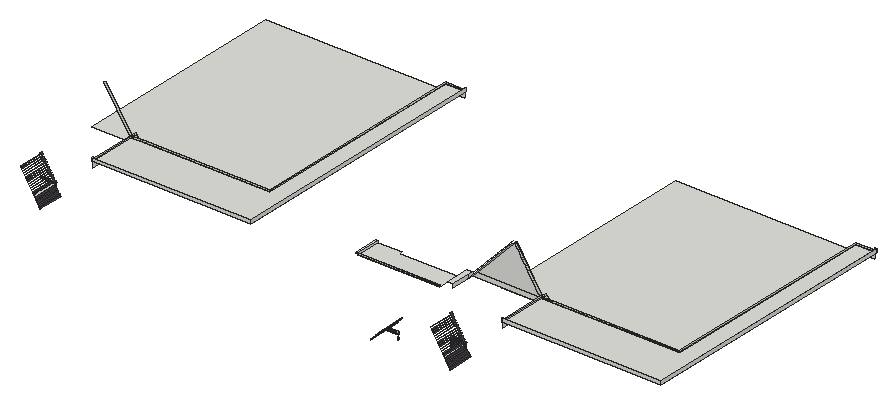
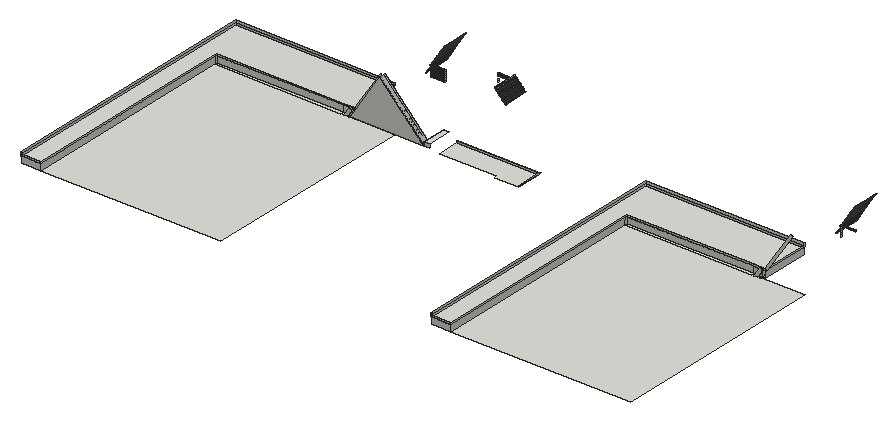
# SketchUp Ruby script. Lengths in inches.
U = 1.inch
M = Sketchup.active_model
def pt(a) = Geom::Point3d.new(a.map { |v| v * U })
def face(e, loops, mat)
  f = e.add_face(loops[0].map { |a| pt(a) })
  loops[1..].each { |l| e.add_face(l.map { |a| pt(a) }).erase! }
  f.material = f.back_material = mat if mat
  f
end
# faces: each face lists its corners as indices into pts; further lists are holes
def faces(e, pts, list, mat = nil) = list.each { |f| face(e, (f[0].is_a?(Array) ? f : [f]).map { |l| l.map { |i| pts[i] } }, mat) }
# xy, xz, yz: faces in a plane at the given z, y or x. An outline is a flat list of corners, or four numbers for a rectangle; further outlines are holes
def ring(l) = l.size == 4 ? [[l[0], l[1]], [l[2], l[1]], [l[2], l[3]], [l[0], l[3]]] : l.each_slice(2).to_a
def flat(e, list, mat, &to3) = list.each { |f| face(e, (f[0].is_a?(Array) ? f : [f]).map { |l| ring(l).map { |u, v| to3.(u, v) } }, mat) }
def xy(e, z, list, mat = nil) = flat(e, list, mat) { |x, y| [x, y, z] }
def xz(e, y, list, mat = nil) = flat(e, list, mat) { |x, z| [x, y, z] }
def yz(e, x, list, mat = nil) = flat(e, list, mat) { |y, z| [x, y, z] }
def lines(e, pts, list) = list.each { |a, b| e.add_line(pt(pts[a]), pt(pts[b])) }
# prism: a flat outline (further loops are holes) pulled along v
def prism(e, loops, v, mat = nil)
  f = face(e, loops, mat); d = Geom::Vector3d.new(v.map { |x| x * U })
  f.pushpull(f.normal.samedirection?(d) ? d.length : -d.length)
end
def box(e, o, s, mat = nil) = prism(e, [[o, [o[0] + s[0], o[1], o[2]], [o[0] + s[0], o[1] + s[1], o[2]], [o[0], o[1] + s[1], o[2]]]], [0, 0, s[2]], mat)
def at(x, y, z, deg = 0) = Geom::Transformation.translation(pt([x, y, z])) * Geom::Transformation.rotation(ORIGIN, Z_AXIS, deg.degrees)
def axes(o, x, y, z) = Geom::Transformation.new([*x, 0, *y, 0, *z, 0, *pt(o).to_a, 1])
def part(name) = M.definitions.add(name)
# library, detail: a bought-in or finely detailed component or shape, given as its bounding box
def library(name, o, s) = part(name).tap { |d| box(d.entities, o, s) }
def detail(e, o, s) = box(e.add_group.entities, o, s)
def put(e, d, t, mat = nil) = e.add_instance(d, t).tap { |i| i.material = mat if mat }
def group(e, t, mat = nil) = e.add_group.tap { |g| g.transformation = t; g.material = mat if mat }.entities
root = M.entities
M.materials.add("[Color M06]").color = [79, 71, 84]
xy(root,341.52,[[2350.98,524.25,2381.95,526.125]])
xy(root,341.93,[[2350.98,524.25,2381.95,526.125]])
xy(root,342.6875,[[2025.57,678.64,2202.51,678.64,2202.51,726.125,2079.13,726.125,2079.13,732.2,2025.57,732.2]])
xy(root,345.06,[[2350.98,524.25,2381.95,526.125]])
xy(root,346,[[2350.98,524.25,2381.95,526.125]])
xy(root,346.3125,[[2023.01,676.08,2025.57,678.64],[2025.57,676.08,2202.51,678.64],[2023.01,678.64,2025.57,732.2]])
xy(root,349.12,[[2350.98,524.25,2381.95,526.125]])
xy(root,350.06,[[2350.98,524.25,2381.95,526.125]])
xy(root,350.1875,[[1523.88,726.125,1797.03,732.2],[2410.35,726.125,2683.5,732.2],[1409.09,732.2,1797.03,1201.875],[2295.55,732.2,2683.5,1201.875]])
xy(root,353.18,[[2350.98,524.25,2381.95,526.125]])
xy(root,354.12,[[2350.98,524.25,2381.95,526.125]])
xy(root,357.25,[[2350.98,524.25,2381.95,526.125]])
xy(root,358.06,[[2350.98,524.25,2381.95,526.125]])
xy(root,358.5,[[2219.8,678.64,2232.12,732.2]])
xy(root,361.18,[[2350.98,524.25,2381.95,526.125]])
xy(root,361.84,[[2244.03,480.14,2246.29,480.77],[2246.89,480.14,2249.21,480.77],[2249.81,480.14,2252.12,480.77],[2252.72,480.14,2255.03,480.77],[2255.63,480.14,2257.94,480.77],
  [2258.54,480.14,2260.86,480.77],[2261.45,480.14,2263.77,480.77],[2264.37,480.14,2266.68,480.77],[2267.28,480.14,2269.59,480.77],[2270.19,480.14,2272.5,480.77]])
xy(root,362,[[2350.98,524.25,2381.95,526.125]])
xy(root,363.75,[[1497.82,620.41,1838.47,623.84],[1838.47,620.41,1841.91,623.84],[2384.28,620.41,2724.93,623.84],[2724.93,620.41,2728.37,623.84],[1497.82,623.84,1497.82,726.125,1797.03,726.125,1797.03,1201.875,1838.47,1201.875,1838.47,623.84],
  [1838.47,623.84,1841.91,1201.875],[2384.28,623.84,2384.28,726.125,2683.5,726.125,2683.5,1201.875,2724.93,1201.875,2724.93,623.84],[2724.93,623.84,2728.37,1201.875]])
xy(root,363.92,[[1495.49,521.5625,1497.36,526.125],[2381.95,521.5625,2383.83,526.125]])
xy(root,364.15,[[2246.2,480.14,2246.29,480.77],[2246.89,480.14,2249.21,480.77],[2249.81,480.14,2252.12,480.77],[2252.72,480.14,2255.03,480.77],[2255.63,480.14,2257.94,480.77],
  [2258.54,480.14,2260.86,480.77],[2261.45,480.14,2263.77,480.77],[2264.37,480.14,2266.68,480.77],[2267.28,480.14,2269.59,480.77],[2270.19,480.14,2272.5,480.77]])
xy(root,364.65,[[2246.89,480.14,2249.21,480.77],[2249.81,480.14,2252.12,480.77],[2252.72,480.14,2255.03,480.77],[2255.63,480.14,2257.94,480.77],[2258.54,480.14,2260.86,480.77],
  [2261.45,480.14,2263.77,480.77],[2264.37,480.14,2266.68,480.77],[2267.28,480.14,2269.59,480.77],[2270.19,480.14,2272.5,480.77]])
xy(root,365.12,[[2350.98,524.25,2381.18,526.125]])
xz(root,480.77,[[2270.19,350.59,2272.5,352.9],[2270.19,353.4,2272.5,355.71]])
xz(root,519.6875,[[1496.99,360.76,1497.36,360.99,1497.31,361.08,1496.9375,360.85],[2383.46,360.76,2383.83,360.99,2383.77,361.08,2383.4,360.85],[1496.3,361.83,1496.67,362.07,1495.49,363.92,1495.49,363.11],[2382.77,361.83,2383.14,362.07,2381.95,363.92,2381.95,363.11],[1495.49,363.11,1495.12,363.68,1495.49,363.92],
  [2381.95,363.11,2381.58,363.68,2381.95,363.92],[1494.67,364.39,1494.61,364.48,1494.98,364.71,1495.04,364.625],[2381.13,364.39,2381.07,364.48,2381.44,364.71,2381.5,364.625]])
xz(root,521.5625,[[2224.98,341.69,2227.4,344.27,2226.95,344.7,2224.53,342.125],[1507.94,343.68,1508.3125,343.92,1506.62,346.56,1506.25,346.32],[2394.41,343.68,2394.77,343.92,2393.08,346.56,2392.71,346.32],[2228.28,345.2,2230.7,347.77,2230.25,348.2,2227.83,345.63],[1505.61,347.3125,1505.98,347.55,1504.29,350.19,1503.92,349.95],
  [2392.08,347.3125,2392.45,347.55,2390.75,350.19,2390.38,349.95],[2231.58,348.7,2234,351.28,2233.55,351.7,2231.125,349.13],[1503.29,350.94,1503.66,351.18,1501.96,353.82,1501.59,353.58],[2389.75,350.94,2390.12,351.18,2388.43,353.82,2388.06,353.58],[2234.88,352.21,2237.3,354.78,2236.84,355.21,2234.42,352.64],
  [1500.96,354.57,1501.33,354.81,1499.63,357.45,1499.27,357.22],[2387.42,354.57,2387.79,354.81,2386.1,357.45,2385.73,357.22],[2238.18,355.71,2240.6,358.28,2240.14,358.71,2237.72,356.14],[1498.63,358.2,1499,358.4375,1497.36,360.99,1497.36,360.18],[2385.1,358.2,2385.46,358.4375,2383.83,360.99,2383.83,360.18],
  [2241.48,359.22,2243.9,361.79,2243.44,362.22,2241.02,359.64],[1497.36,360.18,1496.99,360.76,1497.36,360.99],[2383.83,360.18,2383.46,360.76,2383.83,360.99],[1497.36,360.99,1497.36,363.92,1495.49,363.92,1496.67,362.07,1497.31,361.08],[2383.83,360.99,2383.83,363.92,2381.95,363.92,2383.14,362.07,2383.77,361.08],
  [2244.77,362.72,2247.19,365.29,2246.74,365.72,2244.32,363.15],[1495.12,363.68,1494.67,364.39,1495.04,364.625,1495.49,363.92],[2381.58,363.68,2381.13,364.39,2381.5,364.625,2381.95,363.92],[1493.98,365.46,1492.34,368.02,1492.71,368.25,1494.35,365.7],[2380.44,365.46,2378.8,368.02,2379.17,368.25,2380.81,365.7]])
xz(root,524.25,[[2350.98,341.93,2381.95,345.06],[2350.98,346,2381.95,349.12],[2350.98,350.06,2381.95,353.18],[2350.98,354.12,2381.95,357.25],[2350.98,358.06,2381.95,361.18],
  [1464.52,362,1495.49,362,1495.49,363.92,1494.72,365.12,1464.52,365.12],[2350.98,362,2381.95,362,2381.95,363.92,2381.18,365.12,2350.98,365.12]],"[Color M06]")
xz(root,526.125,[[2350.98,341.52,2381.95,341.93],[2350.98,345.06,2381.95,346],[2350.98,349.12,2381.95,350.06],[2350.98,353.18,2381.95,354.12],[2350.98,357.25,2381.95,358.06],
  [2350.98,361.18,2381.95,362],[1495.49,363.92,1495.49,365.12,1494.72,365.12],[2381.95,363.92,2381.95,365.12,2381.18,365.12],[2350.98,365.12,2381.18,365.12,2380.46,366.25,2350.98,366.25]])
xz(root,620.41,[[1497.82,363.75,1841.91,370.8125],[2384.28,363.75,2728.37,370.8125]])
xz(root,623.84,[[1497.82,363.75,1838.47,367.1875],[2384.28,363.75,2724.93,367.1875]])
xz(root,678.64,[[2025.57,342.6875,2202.51,346.3125]])
xz(root,726.125,[[1497.82,350.1875,1497.82,360.28,1504.29,350.1875],[1504.29,350.1875,1504.29,359.1,1501.3125,363.75,1497.82,363.75,1497.82,360.28],[1504.29,350.1875,1510.01,350.1875,1504.29,359.1],[1510.01,350.1875,1504.29,359.1,1504.29,363.75,1510.01,363.75],[1510.01,350.1875,1523.88,363.75],
  [1523.88,350.1875,1797.03,363.75],[2384.28,350.1875,2384.28,360.28,2390.75,350.1875],[2390.75,350.1875,2390.75,359.1,2387.78,363.75,2384.28,363.75,2384.28,360.28],[2390.75,350.1875,2396.47,350.1875,2390.75,359.1],[2396.47,350.1875,2390.75,359.1,2390.75,363.75,2396.47,363.75],
  [2396.47,350.1875,2410.35,363.75],[2410.35,350.1875,2683.5,363.75],[1504.29,359.1,1501.3125,363.75,1504.29,363.75],[2390.75,359.1,2387.78,363.75,2390.75,363.75],[1497.82,360.28,1497.82,364.9375,1494.83,364.9375],
  [2384.28,360.28,2384.28,364.9375,2381.3,364.9375],[1497.82,363.75,1497.82,364.9375,1500.55,364.9375,1501.3125,363.75],[1501.3125,363.75,1500.55,364.9375,1499.11,367.1875,1501.3125,367.1875],[1501.3125,363.75,1504.29,367.1875],[1504.29,363.75,1510.01,367.1875],
  [1510.01,363.75,1523.88,367.1875],[1523.88,363.75,1797.03,367.1875],[2384.28,363.75,2384.28,364.9375,2387.01,364.9375,2387.78,363.75],[2387.78,363.75,2387.01,364.9375,2385.57,367.1875,2387.78,367.1875],[2387.78,363.75,2390.75,367.1875],
  [2390.75,363.75,2396.47,367.1875],[2396.47,363.75,2410.35,367.1875],[2410.35,363.75,2683.5,367.1875],[1494.83,364.9375,1440.02,450.4375,1444.07,453.03,1498.89,367.53,1498.34,367.1875,1497.82,367.1875,1497.82,366.85],[1494.83,364.9375,1497.82,366.85,1497.82,364.9375],
  [1497.82,364.9375,1497.82,366.85,1498.34,367.1875,1499.11,367.1875,1500.55,364.9375],[2246,364.9375,2326.48,450.4375,2381.3,364.9375],[2381.3,364.9375,2326.48,450.4375,2330.53,453.03,2385.35,367.53,2384.81,367.1875,2384.28,367.1875,2384.28,366.85],[2381.3,364.9375,2384.28,366.85,2384.28,364.9375],[2384.28,364.9375,2384.28,366.85,2384.81,367.1875,2385.57,367.1875,2387.01,364.9375]])
xz(root,731.75,[[2219.8,357.04,2219.08,357.73,2219.8,358.5]])
xz(root,732.2,[[1517.43,340.75,1521.72,343.5,1517.43,350.1875],[2403.9,340.75,2408.18,343.5,2403.9,350.1875],[1510.01,341.27,1510.01,350.1875,1504.29,350.1875],[2396.47,341.27,2396.47,350.1875,2390.75,350.1875],[1510.01,350.1875,1500.55,364.9375,1505.8125,368.3125,1517.43,350.1875],
  [2219.8,350.1875,2232.12,358.5],[2232.12,350.1875,2326.48,450.4375,2390.75,350.1875],[2396.47,350.1875,2387.01,364.9375,2392.28,368.3125,2403.9,350.1875],[1500.55,364.9375,1498.89,367.53,1504.15,370.91,1505.8125,368.3125],[2387.01,364.9375,2385.35,367.53,2390.61,370.91,2392.28,368.3125]])
xz(root,1201.875,[[1797.03,350.1875,1838.47,363.75],[2683.5,350.1875,2724.93,363.75],[1797.03,363.75,1838.47,367.1875],[1838.47,363.75,1841.91,370.8125],[2683.5,363.75,2724.93,367.1875],
  [2724.93,363.75,2728.37,370.8125]])
yz(root,1495.49,[[524.25,341.93,526.125,345.06],[524.25,346,526.125,349.12],[524.25,350.06,526.125,353.18],[524.25,354.12,526.125,357.25],[524.25,358.06,526.125,361.18],
  [524.25,362,526.125,363.92]])
yz(root,1497.82,[[623.84,350.1875,726.125,363.75],[620.41,363.75,623.84,370.8125],[623.84,363.75,726.125,367.1875]])
yz(root,1797.03,[[726.125,350.1875,732.2,363.75],[732.2,350.1875,1201.875,363.75],[726.125,363.75,732.2,367.1875],[732.2,363.75,1201.875,367.1875]])
yz(root,1838.47,[[623.84,363.75,1201.875,367.1875]])
yz(root,1841.91,[[620.41,363.75,1201.875,370.8125]])
yz(root,2025.57,[[678.64,342.6875,732.2,346.3125]])
yz(root,2232.12,[[678.64,350.1875,719.59,358.5],[719.59,350.1875,731.75,358.5],[731.75,350.1875,732.2,358.5]])
yz(root,2246.29,[[480.14,361.84,480.77,364.15]])
yz(root,2246.89,[[480.14,361.84,480.77,364.15],[480.14,364.65,480.77,364.89]])
yz(root,2249.21,[[480.14,361.84,480.77,364.15],[480.14,364.65,480.77,366.96]])
yz(root,2249.81,[[480.14,361.84,480.77,364.15],[480.14,364.65,480.77,366.96]])
yz(root,2252.12,[[480.14,361.84,480.77,364.15],[480.14,364.65,480.77,366.96]])
yz(root,2252.72,[[480.14,361.84,480.77,364.15],[480.14,364.65,480.77,366.96]])
yz(root,2255.03,[[480.14,361.84,480.77,364.15],[480.14,364.65,480.77,366.96]])
yz(root,2255.63,[[480.14,361.84,480.77,364.15],[480.14,364.65,480.77,366.96]])
yz(root,2257.94,[[480.14,361.84,480.77,364.15],[480.14,364.65,480.77,366.96]])
yz(root,2258.54,[[480.14,361.84,480.77,364.15],[480.14,364.65,480.77,366.96]])
yz(root,2260.86,[[480.14,361.84,480.77,364.15],[480.14,364.65,480.77,366.96]])
yz(root,2261.45,[[480.14,361.84,480.77,364.15],[480.14,364.65,480.77,366.96]])
yz(root,2263.77,[[480.14,361.84,480.77,364.15],[480.14,364.65,480.77,366.96]])
yz(root,2264.37,[[480.14,364.65,480.77,366.96]])
yz(root,2266.68,[[480.14,361.84,480.77,364.15],[480.14,364.65,480.77,366.96]])
yz(root,2267.28,[[480.14,361.84,480.77,364.15],[480.14,364.65,480.77,366.96]])
yz(root,2269.59,[[480.14,361.84,480.77,364.15],[480.14,364.65,480.77,366.96]])
yz(root,2270.19,[[480.14,361.84,480.77,364.15],[480.14,364.65,480.77,366.96]])
yz(root,2272.5,[[480.14,361.84,480.77,364.15],[480.14,364.65,480.77,366.96]])
yz(root,2350.98,[[524.25,341.93,526.125,345.06],[524.25,346,526.125,349.12],[524.25,350.06,526.125,353.18],[524.25,354.12,526.125,357.25],[524.25,358.06,526.125,361.18],
  [524.25,362,526.125,365.12]])
yz(root,2381.95,[[524.25,341.93,526.125,345.06],[524.25,346,526.125,349.12],[524.25,350.06,526.125,353.18],[524.25,354.12,526.125,357.25],[524.25,358.06,526.125,361.18],
  [524.25,362,526.125,363.92]])
yz(root,2384.28,[[623.84,350.1875,726.125,363.75],[620.41,363.75,623.84,370.8125],[623.84,363.75,726.125,367.1875]])
yz(root,2683.5,[[726.125,350.1875,732.2,363.75],[732.2,350.1875,1201.875,363.75],[726.125,363.75,732.2,367.1875],[732.2,363.75,1201.875,367.1875]])
yz(root,2724.93,[[623.84,363.75,1201.875,367.1875]])
yz(root,2728.37,[[620.41,363.75,1201.875,370.8125]])
p = [[2223.65,521.5625,341.19],[2223.65,467.1875,341.19],[2224.11,467.1875,340.76],[2224.11,521.5625,340.76],[2224.53,521.5625,342.125],[2224.53,467.1875,342.125],
  [2224.98,521.5625,341.69],[2224.98,467.1875,341.69],[2227.4,521.5625,344.27],[2227.4,467.1875,344.27],[1508.94,467.1875,342.93],[1508.94,521.5625,342.93],
  [1508.58,521.5625,342.69],[1508.58,467.1875,342.69],[2395.41,467.1875,342.93],[2395.41,521.5625,342.93],[2395.04,521.5625,342.69],[2395.04,467.1875,342.69],
  [1508.3125,467.1875,343.92],[1508.3125,521.5625,343.92],[2394.77,467.1875,343.92],[2394.77,521.5625,343.92],[1506.25,521.5625,346.32],[1507.94,521.5625,343.68],
  [1507.94,467.1875,343.68],[1506.25,467.1875,346.32],[2392.71,521.5625,346.32],[2394.41,521.5625,343.68],[2394.41,467.1875,343.68],[2392.71,467.1875,346.32],
  [2226.95,521.5625,344.7],[2226.95,467.1875,344.7],[2227.83,521.5625,345.63],[2227.83,467.1875,345.63],[2228.28,521.5625,345.2],[2228.28,467.1875,345.2],
  [2230.7,521.5625,347.77],[2230.7,467.1875,347.77],[1506.62,467.1875,346.56],[1506.62,521.5625,346.56],[2393.08,467.1875,346.56],[2393.08,521.5625,346.56],
  [1505.98,467.1875,347.55],[1505.98,521.5625,347.55],[2392.45,467.1875,347.55],[2392.45,521.5625,347.55],[1503.92,521.5625,349.95],[1505.61,521.5625,347.3125],
  [1505.61,467.1875,347.3125],[1503.92,467.1875,349.95],[2390.38,521.5625,349.95],[2392.08,521.5625,347.3125],[2392.08,467.1875,347.3125],[2390.38,467.1875,349.95],
  [2230.25,521.5625,348.2],[2230.25,467.1875,348.2],[2231.125,521.5625,349.13],[2231.125,467.1875,349.13],[2231.58,521.5625,348.7],[2231.58,467.1875,348.7],
  [2234,521.5625,351.28],[2234,467.1875,351.28],[1504.29,467.1875,350.19],[1504.29,521.5625,350.19],[2390.75,467.1875,350.19],[2390.75,521.5625,350.19],
  [1503.66,467.1875,351.18],[1503.66,521.5625,351.18],[2390.12,467.1875,351.18],[2390.12,521.5625,351.18],[2326.48,731.75,450.4375],[2232.12,731.75,350.1875],
  [2232.12,719.59,350.1875],[2326.48,719.59,450.4375],[2326.48,726.125,450.4375],[2326.48,732.2,450.4375],[2232.12,732.2,350.1875],[1501.59,521.5625,353.58],
  [1503.29,521.5625,350.94],[1503.29,467.1875,350.94],[1501.59,467.1875,353.58],[2388.06,521.5625,353.58],[2389.75,521.5625,350.94],[2389.75,467.1875,350.94],
  [2388.06,467.1875,353.58],[2233.55,521.5625,351.7],[2233.55,467.1875,351.7],[2234.42,521.5625,352.64],[2234.42,467.1875,352.64],[2234.88,521.5625,352.21],
  [2234.88,467.1875,352.21],[2237.3,521.5625,354.78],[2237.3,467.1875,354.78],[1501.96,467.1875,353.82],[1501.96,521.5625,353.82],[2388.43,467.1875,353.82],
  [2388.43,521.5625,353.82],[1501.33,467.1875,354.81],[1501.33,521.5625,354.81],[2387.79,467.1875,354.81],[2387.79,521.5625,354.81],[1499.27,521.5625,357.22],
  [1500.96,521.5625,354.57],[1500.96,467.1875,354.57],[1499.27,467.1875,357.22],[2385.73,521.5625,357.22],[2387.42,521.5625,354.57],[2387.42,467.1875,354.57],
  [2385.73,467.1875,357.22],[2236.84,521.5625,355.21],[2236.84,467.1875,355.21],[2237.72,521.5625,356.14],[2237.72,467.1875,356.14],[2238.18,521.5625,355.71],
  [2238.18,480.14,355.71],[2238.18,467.1875,355.71],[2240.6,521.5625,358.28],[2240.6,467.1875,358.28],[1499.63,467.1875,357.45],[1499.63,521.5625,357.45],
  [2386.1,467.1875,357.45],[2386.1,521.5625,357.45],[1499,467.1875,358.4375],[1499,521.5625,358.4375],[2385.46,467.1875,358.4375],[2385.46,521.5625,358.4375],
  [1496.9375,467.1875,360.85],[1496.9375,519.6875,360.85],[1496.99,519.6875,360.76],[1496.99,521.5625,360.76],[1497.36,521.5625,360.18],[1498.63,521.5625,358.2],
  [1498.63,467.1875,358.2],[2383.4,467.1875,360.85],[2383.4,519.6875,360.85],[2383.46,519.6875,360.76],[2383.46,521.5625,360.76],[2383.83,521.5625,360.18],
  [2385.1,521.5625,358.2],[2385.1,467.1875,358.2],[2240.14,521.5625,358.71],[2240.14,467.1875,358.71],[2241.02,521.5625,359.64],[2241.02,467.1875,359.64],
  [2241.48,521.5625,359.22],[2241.48,467.1875,359.22],[2243.9,521.5625,361.79],[2243.9,467.1875,361.79],[1497.31,467.1875,361.08],[1497.31,519.6875,361.08],
  [2383.77,467.1875,361.08],[2383.77,519.6875,361.08],[1497.36,519.6875,360.99],[1497.36,521.5625,360.99],[2383.83,519.6875,360.99],[2383.83,521.5625,360.99],
  [1497.31,521.5625,361.08],[2383.77,521.5625,361.08],[1496.67,467.1875,362.07],[1496.67,519.6875,362.07],[2383.14,467.1875,362.07],[2383.14,519.6875,362.07],
  [1496.67,521.5625,362.07],[2383.14,521.5625,362.07],[1494.61,467.1875,364.48],[1494.61,519.6875,364.48],[1494.67,519.6875,364.39],[1494.67,521.5625,364.39],
  [1495.12,521.5625,363.68],[1495.12,519.6875,363.68],[1495.49,519.6875,363.11],[1496.3,519.6875,361.83],[1496.3,467.1875,361.83],[2243.44,521.5625,362.22],
  [2243.44,467.1875,362.22],[2381.07,467.1875,364.48],[2381.07,519.6875,364.48],[2381.13,519.6875,364.39],[2381.13,521.5625,364.39],[2381.58,521.5625,363.68],
  [2381.58,519.6875,363.68],[2381.95,519.6875,363.11],[2382.77,519.6875,361.83],[2382.77,467.1875,361.83],[2246.2,480.14,364.15],[2244.03,480.14,361.84],
  [2244.03,480.77,361.84],[2246.2,480.77,364.15],[1494.98,467.1875,364.71],[1494.98,519.6875,364.71],[1494.98,521.5625,364.71],[1495.04,521.5625,364.625],
  [1495.49,521.5625,363.92],[1495.49,519.6875,363.92],[2381.44,467.1875,364.71],[2381.44,519.6875,364.71],[2381.44,521.5625,364.71],[2381.5,521.5625,364.625],
  [2381.95,521.5625,363.92],[2381.95,519.6875,363.92],[2244.32,521.5625,363.15],[2244.32,467.1875,363.15],[2244.77,521.5625,362.72],[2244.77,467.1875,362.72],
  [2247.19,521.5625,365.29],[2247.19,467.1875,365.29],[1495.49,524.25,363.92],[1494.35,467.1875,365.7],[1494.35,521.5625,365.7],[1492.71,521.5625,368.25],
  [1492.71,519.6875,368.25],[1492.65,519.6875,368.34],[1492.65,467.1875,368.34],[1492.02,467.1875,369.33],[1492.02,521.5625,369.33],[1490.38,521.5625,371.88],
  [1490.38,519.6875,371.88],[1490.32,519.6875,371.97],[1490.32,467.1875,371.97],[1489.83,467.1875,372.75],[1489.83,521.5625,372.75],[1488.1875,521.5625,375.3],
  [1488.1875,519.6875,375.3],[1488.13,519.6875,375.39],[1488.13,467.1875,375.39],[1487.63,467.1875,376.17],[1487.63,521.5625,376.17],[1485.99,521.5625,378.72],
  [1485.99,519.6875,378.72],[1485.9375,519.6875,378.8125],[1485.9375,467.1875,378.8125],[1485.44,467.1875,379.59],[1485.44,521.5625,379.59],[1483.8,521.5625,382.14],
  [1483.8,519.6875,382.14],[1483.75,519.6875,382.23],[1483.75,467.1875,382.23],[1483.25,467.1875,383.01],[1483.25,521.5625,383.01],[1481.61,521.5625,385.56],
  [1481.61,519.6875,385.56],[1481.55,519.6875,385.65],[1481.55,467.1875,385.65],[1481.05,467.1875,386.43],[1481.05,521.5625,386.43],[1479.42,521.5625,388.98],
  [1479.42,519.6875,388.98],[1479.36,519.6875,389.07],[1479.36,467.1875,389.07],[1478.86,467.1875,389.85],[1478.86,521.5625,389.85],[1477.22,521.5625,392.4],
  [1477.22,519.6875,392.4],[1477.17,519.6875,392.49],[1477.17,467.1875,392.49],[1476.67,467.1875,393.27],[1476.67,521.5625,393.27],[1475.03,521.5625,395.82],
  [1475.03,519.6875,395.82],[1474.98,519.6875,395.91],[1474.98,467.1875,395.91],[1474.48,467.1875,396.69],[1474.48,521.5625,396.69],[1472.84,521.5625,399.24],
  [1472.84,519.6875,399.24],[1472.78,519.6875,399.33],[1472.78,467.1875,399.33],[1472.28,467.1875,400.11],[1472.28,521.5625,400.11],[1470.65,521.5625,402.66],
  [1470.65,519.6875,402.66],[1470.59,519.6875,402.75],[1470.59,467.1875,402.75],[1470.09,467.1875,403.53],[1470.09,521.5625,403.53],[1468.45,521.5625,406.08],
  [1468.45,519.6875,406.08],[1468.4,519.6875,406.17],[1468.4,467.1875,406.17],[1467.9,467.1875,406.95],[1467.9,521.5625,406.95],[1466.26,521.5625,409.5],
  [1466.26,519.6875,409.5],[1466.2,519.6875,409.59],[1466.2,467.1875,409.59],[1465.71,467.1875,410.37],[1465.71,521.5625,410.37],[1464.52,521.5625,412.22],
  [1464.52,526.125,412.22],[1464.58,526.125,412.12],[1466.59,526.125,409],[1467.47,526.125,407.62],[1467.47,524.25,407.62],[1469.47,524.25,404.5],
  [1469.47,526.125,404.5],[1470.19,526.125,403.37],[1470.19,524.25,403.37],[1472.2,524.25,400.25],[1472.2,526.125,400.25],[1472.92,526.125,399.12],
  [1472.92,524.25,399.12],[1474.92,524.25,396],[1474.92,526.125,396],[1475.64,526.125,394.87],[1475.64,524.25,394.87],[1477.65,524.25,391.75],
  [1477.65,526.125,391.75],[1478.37,526.125,390.62],[1478.37,524.25,390.62],[1480.37,524.25,387.5],[1480.37,526.125,387.5],[1481.09,526.125,386.37],
  [1481.09,524.25,386.37],[1483.1,524.25,383.25],[1483.1,526.125,383.25],[1483.82,526.125,382.12],[1483.82,524.25,382.12],[1485.82,524.25,379],
  [1485.82,526.125,379],[1486.54,526.125,377.87],[1486.54,524.25,377.87],[1488.55,524.25,374.75],[1488.55,526.125,374.75],[1489.27,526.125,373.62],
  [1489.27,524.25,373.62],[1491.27,524.25,370.5],[1491.27,526.125,370.5],[1491.99,526.125,369.37],[1491.99,524.25,369.37],[1494,524.25,366.25],
  [1494,526.125,366.25],[1494.72,526.125,365.12],[1494.72,524.25,365.12],[2381.95,524.25,363.92],[2380.81,467.1875,365.7],[2380.81,521.5625,365.7],
  [2379.17,521.5625,368.25],[2379.17,519.6875,368.25],[2379.11,519.6875,368.34],[2379.11,467.1875,368.34],[2378.48,467.1875,369.33],[2378.48,521.5625,369.33],
  [2376.84,521.5625,371.88],[2376.84,519.6875,371.88],[2376.79,519.6875,371.97],[2376.79,467.1875,371.97],[2376.29,467.1875,372.75],[2376.29,521.5625,372.75],
  [2374.65,521.5625,375.3],[2374.65,519.6875,375.3],[2374.59,519.6875,375.39],[2374.59,467.1875,375.39],[2374.1,467.1875,376.17],[2374.1,521.5625,376.17],
  [2372.46,521.5625,378.72],[2372.46,519.6875,378.72],[2372.4,519.6875,378.8125],[2372.4,467.1875,378.8125],[2371.9,467.1875,379.59],[2371.9,521.5625,379.59],
  [2370.27,521.5625,382.14],[2370.27,519.6875,382.14],[2370.21,519.6875,382.23],[2370.21,467.1875,382.23],[2369.71,467.1875,383.01],[2369.71,521.5625,383.01],
  [2368.07,521.5625,385.56],[2368.07,519.6875,385.56],[2368.02,519.6875,385.65],[2368.02,467.1875,385.65],[2367.52,467.1875,386.43],[2367.52,521.5625,386.43],
  [2365.88,521.5625,388.98],[2365.88,519.6875,388.98],[2365.82,519.6875,389.07],[2365.82,467.1875,389.07],[2365.33,467.1875,389.85],[2365.33,521.5625,389.85],
  [2363.6875,521.5625,392.4],[2363.6875,519.6875,392.4],[2363.63,519.6875,392.49],[2363.63,467.1875,392.49],[2363.13,467.1875,393.27],[2363.13,521.5625,393.27],
  [2361.5,521.5625,395.82],[2361.5,519.6875,395.82],[2361.4375,519.6875,395.91],[2361.4375,467.1875,395.91],[2360.94,467.1875,396.69],[2360.94,521.5625,396.69],
  [2359.3,521.5625,399.24],[2359.3,519.6875,399.24],[2359.25,519.6875,399.33],[2359.25,467.1875,399.33],[2358.75,467.1875,400.11],[2358.75,521.5625,400.11],
  [2357.11,521.5625,402.66],[2357.11,519.6875,402.66],[2357.05,519.6875,402.75],[2357.05,467.1875,402.75],[2356.56,467.1875,403.53],[2356.56,521.5625,403.53],
  [2354.92,521.5625,406.08],[2354.92,519.6875,406.08],[2354.86,519.6875,406.17],[2354.86,467.1875,406.17],[2354.36,467.1875,406.95],[2354.36,521.5625,406.95],
  [2352.73,521.5625,409.5],[2352.73,519.6875,409.5],[2352.67,519.6875,409.59],[2352.67,467.1875,409.59],[2352.17,467.1875,410.37],[2352.17,521.5625,410.37],
  [2350.98,521.5625,412.22],[2350.98,526.125,412.22],[2351.05,526.125,412.12],[2353.05,526.125,409],[2353.93,526.125,407.62],[2353.93,524.25,407.62],
  [2355.9375,524.25,404.5],[2355.9375,526.125,404.5],[2356.66,526.125,403.37],[2356.66,524.25,403.37],[2358.66,524.25,400.25],[2358.66,526.125,400.25],
  [2359.38,526.125,399.12],[2359.38,524.25,399.12],[2361.39,524.25,396],[2361.39,526.125,396],[2362.11,526.125,394.87],[2362.11,524.25,394.87],
  [2364.11,524.25,391.75],[2364.11,526.125,391.75],[2364.83,526.125,390.62],[2364.83,524.25,390.62],[2366.84,524.25,387.5],[2366.84,526.125,387.5],
  [2367.56,526.125,386.37],[2367.56,524.25,386.37],[2369.5625,524.25,383.25],[2369.5625,526.125,383.25],[2370.28,526.125,382.12],[2370.28,524.25,382.12],
  [2372.29,524.25,379],[2372.29,526.125,379],[2373.01,526.125,377.87],[2373.01,524.25,377.87],[2375.01,524.25,374.75],[2375.01,526.125,374.75],
  [2375.73,526.125,373.62],[2375.73,524.25,373.62],[2377.73,524.25,370.5],[2377.73,526.125,370.5],[2378.45,526.125,369.37],[2378.45,524.25,369.37],
  [2380.46,524.25,366.25],[2380.46,526.125,366.25],[2381.18,526.125,365.12],[2381.18,524.25,365.12],[1495.49,526.125,363.92],[2381.95,526.125,363.92],
  [1495.04,519.6875,364.625],[2381.5,519.6875,364.625],[2248.83,480.14,366.96],[2246.89,480.14,364.89],[2246.89,480.77,364.89],[2248.83,480.77,366.96],
  [1499.11,726.125,367.1875],[1498.89,726.125,367.53],[1498.89,732.2,367.53],[1500.55,732.2,364.9375],[1500.55,726.125,364.9375],[2385.57,726.125,367.1875],
  [2385.35,726.125,367.53],[2385.35,732.2,367.53],[2387.01,732.2,364.9375],[2387.01,726.125,364.9375],[2246.74,521.5625,365.72],[2246.74,467.1875,365.72],
  [1492.28,467.1875,368.11],[1492.28,519.6875,368.11],[1492.34,519.6875,368.02],[1492.34,521.5625,368.02],[1493.98,521.5625,365.46],[1493.98,467.1875,365.46],
  [2378.75,467.1875,368.11],[2378.75,519.6875,368.11],[2378.8,519.6875,368.02],[2378.8,521.5625,368.02],[2380.44,521.5625,365.46],[2380.44,467.1875,365.46],
  [2247.62,521.5625,366.65],[2247.62,467.1875,366.65],[2240.08,726.125,364.9375],[2323.29,726.125,453.34],[2219.8,731.75,358.5],[2220.53,731.75,357.81]]
faces(root,p,[[0,1,2,3],[10,11,12,13],[14,15,16,17],[19,18,24,23],[21,20,28,27],[33,32,34,35],[38,39,22,25],[40,41,26,29],
  [43,42,48,47],[45,44,52,51],[57,56,58,59],[62,63,46,49],[64,65,50,53],[70,71,72,73,74],[75,76,71,70],[67,66,79,78],
  [69,68,83,82],[88,87,89,90],[93,94,77,80],[95,96,81,84],[98,97,103,102],[100,99,107,106],[112,111,113,114,115],[118,119,101,104],
  [120,121,105,108],[123,122,132,131],[125,124,139,138],[143,142,144,145],[148,149,127,126],[150,151,134,133],[152,153,129,128],[154,155,136,135],
  [152,149,156,153],[154,151,157,155],[149,159,162,156],[151,161,163,157],[159,158,172,171],[161,160,183,182],[184,185,186,187],[158,188,189,190,191,192,193,159],
  [160,194,195,196,197,198,199,161],[192,162,159,193],[198,163,161,199],[201,200,202,203],[192,193,169,168],[198,199,180,179],[331,460,206,332],[458,461,333,459],
  [462,191,167,166],[463,197,178,177],[188,189,165,164],[194,195,176,175],[464,465,466,467],[468,469,470,471,472],[473,474,475,476,477],[478,479,205,204],
  [208,207,485,484],[335,334,491,490]])
faces(root,p,[[0,4,5,1],[5,4,6,7],[6,8,9,7],[10,18,19,11],[14,20,21,15],[22,23,24,25],[26,27,28,29],[30,31,9,8],
  [30,32,33,31],[34,36,37,35],[38,42,43,39],[40,44,45,41],[46,47,48,49],[50,51,52,53],[54,55,37,36],[54,56,57,55],
  [58,60,61,59],[62,66,67,63],[64,68,69,65],[77,78,79,80],[81,82,83,84],[85,86,61,60],[85,87,88,86],[89,91,92,90],
  [93,97,98,94],[95,99,100,96],[101,102,103,104],[105,106,107,108],[109,110,92,91],[109,111,112,110],[113,116,117,115,114],[118,122,123,119],
  [120,124,125,121],[126,127,128,129,130,131,132],[133,134,135,136,137,138,139],[140,141,117,116],[140,142,143,141],[144,146,147,145],[148,158,159,149],[150,160,161,151],
  [164,165,166,167,168,169,170,171,172],[173,174,147,146],[175,176,177,178,179,180,181,182,183],[173,200,201,174],[202,204,205,203],[206,192,191,190,189,188,207,208,209,210,211,212,213,214,215,216,217,218,219,220,221,222,223,224,225,226,227,228,229,230,231,232,233,234,235,236,237,238,239,240,241,242,243,244,245,246,247,248,249,250,251,252,253,254,255,256,257,258,259,260,261,262,263,264,265,266,267,268,269,270,271,272,273,274,275,276,277,278,279,280,281,282,283,284,285,286,287,288,289,290,291,292,293,294,295,296,297,298,299,300,301,302,303,304,305,306,307,308,309,310,311,312,313,314,315,316,317,318,319,320,321,322,323,324,325,326,327,328,329,330,331,332],[333,198,197,196,195,194,334,335,336,337,338,339,340,341,342,343,344,345,346,347,348,349,350,351,352,353,354,355,356,357,358,359,360,361,362,363,364,365,366,367,368,369,370,371,372,373,374,375,376,377,378,379,380,381,382,383,384,385,386,387,388,389,390,391,392,393,394,395,396,397,398,399,400,401,402,403,404,405,406,407,408,409,410,411,412,413,414,415,416,417,418,419,420,421,422,423,424,425,426,427,428,429,430,431,432,433,434,435,436,437,438,439,440,441,442,443,444,445,446,447,448,449,450,451,452,453,454,455,456,457,458,459],[480,481,482,483,484,485],
  [486,487,488,489,490,491],[478,492,493,479]],"[Color M06]")
lines(root,p,[[494,495],[496,497]])
